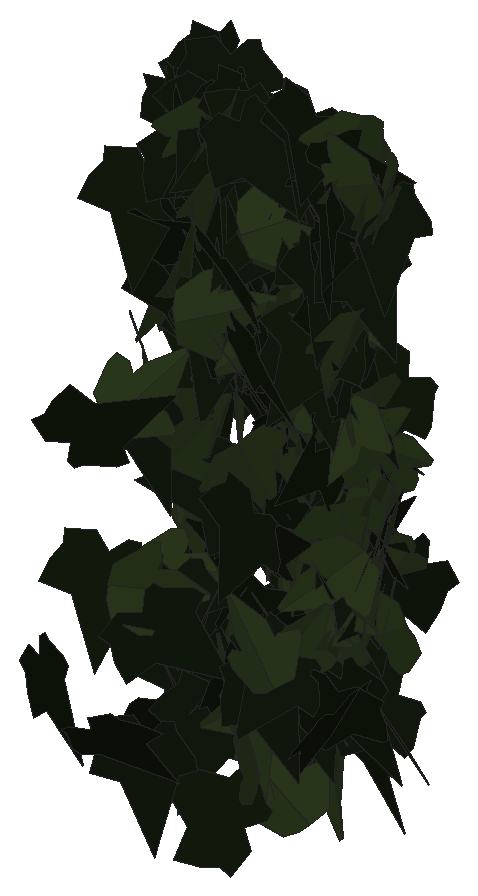
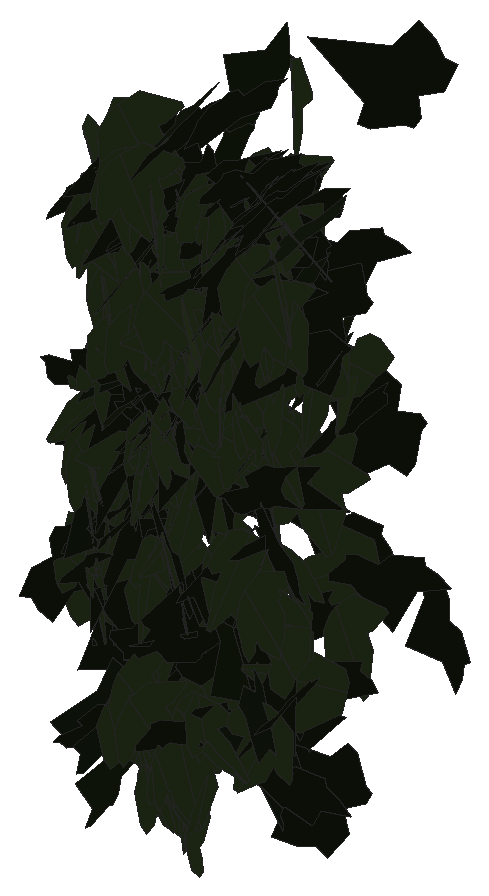
# SketchUp Ruby script. Lengths in inches.
U = 1.inch
M = Sketchup.active_model
def pt(a) = Geom::Point3d.new(a.map { |v| v * U })
def face(e, loops, mat)
  f = e.add_face(loops[0].map { |a| pt(a) })
  loops[1..].each { |l| e.add_face(l.map { |a| pt(a) }).erase! }
  f.material = f.back_material = mat if mat
  f
end
# faces: each face lists its corners as indices into pts; further lists are holes
def faces(e, pts, list, mat = nil) = list.each { |f| face(e, (f[0].is_a?(Array) ? f : [f]).map { |l| l.map { |i| pts[i] } }, mat) }
# xy, xz, yz: faces in a plane at the given z, y or x. An outline is a flat list of corners, or four numbers for a rectangle; further outlines are holes
def ring(l) = l.size == 4 ? [[l[0], l[1]], [l[2], l[1]], [l[2], l[3]], [l[0], l[3]]] : l.each_slice(2).to_a
def flat(e, list, mat, &to3) = list.each { |f| face(e, (f[0].is_a?(Array) ? f : [f]).map { |l| ring(l).map { |u, v| to3.(u, v) } }, mat) }
def xy(e, z, list, mat = nil) = flat(e, list, mat) { |x, y| [x, y, z] }
def xz(e, y, list, mat = nil) = flat(e, list, mat) { |x, z| [x, y, z] }
def yz(e, x, list, mat = nil) = flat(e, list, mat) { |y, z| [x, y, z] }
def lines(e, pts, list) = list.each { |a, b| e.add_line(pt(pts[a]), pt(pts[b])) }
# prism: a flat outline (further loops are holes) pulled along v
def prism(e, loops, v, mat = nil)
  f = face(e, loops, mat); d = Geom::Vector3d.new(v.map { |x| x * U })
  f.pushpull(f.normal.samedirection?(d) ? d.length : -d.length)
end
def box(e, o, s, mat = nil) = prism(e, [[o, [o[0] + s[0], o[1], o[2]], [o[0] + s[0], o[1] + s[1], o[2]], [o[0], o[1] + s[1], o[2]]]], [0, 0, s[2]], mat)
def at(x, y, z, deg = 0) = Geom::Transformation.translation(pt([x, y, z])) * Geom::Transformation.rotation(ORIGIN, Z_AXIS, deg.degrees)
def axes(o, x, y, z) = Geom::Transformation.new([*x, 0, *y, 0, *z, 0, *pt(o).to_a, 1])
def part(name) = M.definitions.add(name)
# library, detail: a bought-in or finely detailed component or shape, given as its bounding box
def library(name, o, s) = part(name).tap { |d| box(d.entities, o, s) }
def detail(e, o, s) = box(e.add_group.entities, o, s)
def put(e, d, t, mat = nil) = e.add_instance(d, t).tap { |i| i.material = mat if mat }
def group(e, t, mat = nil) = e.add_group.tap { |g| g.transformation = t; g.material = mat if mat }.entities
root = M.entities
M.materials.add("efeu1").color = [18, 25, 13]
M.materials.add("efeu2").color = [43, 57, 29]
c1 = part("ivyleaf_9")
p = [[1.54,2.16,1.25],[1.36,2.04,1.19],[-0.21,0.99,0.68],[-0.71,1.11,0.82],[-0.85,0.86,0.67],[-0.8,0.17,0.21],
  [-0.9,-0.01,0.1],[-0.67,-0.16,-0.02],[-0.08,-0.08,-0.05],[-0.03,-0.6,-0.4],[0.65,-0.88,-0.66],[0.83,-0.6,-0.49],
  [1.29,-0.42,-0.43],[1.8125,-0.07,-0.26],[1.21,0.44,0.15]]
faces(c1.entities,p,[[0,1,2,3,4,5,6,7,8,9,10,11,12,13,14]],"efeu1")
c2 = part("ivyleaf_10")
p = [[0,0.5,-0.03],[-0.0625,2.02,-0.43],[-0.19,2.01,-0.46],[-0.54,1.05,-0.29],[-0.52,0.625,-0.18],[-0.83,0.76,-0.28],
  [-1.16,0.64,-0.33],[-1.15,0.33,-0.24],[-0.77,-0.39,0.02],[-0.3,-0.51,0.16],[0.04,-0.48,0.23],[-0.02,2.01,-0.4375],
  [-0.06,2.01,-0.43],[0.04,-0.49,0.23],[0.67,-0.49,0.14],[1.38,0.36,-0.2],[1.375,0.51,-0.24],[0.81,0.65,-0.19],
  [0.62,0.59,-0.15],[0.6,1.09,-0.28],[0.5,1.23,-0.31]]
faces(c2.entities,p,[[0,1,2,3,4,5,6,7,8,9,10],[11,12,0,13,14,15,16,17,18,19,20]],"efeu2")
put(root,c1,axes([15.72,223.31,221.94],[-0.24681,-0.41121,-0.14139],[0.07625,0.11913,-0.47958],[0.4281,-0.25829,0.0039]))
put(root,c1,axes([16.01,224.52,223.05],[-0.47711,0.12724,-0.07858],[0.06987,-0.04261,-0.49326],[-0.13223,-0.48166,0.02288]))
put(root,c1,axes([15.53,224.26,222.49],[0.09405,-0.47818,0.11179],[0.14245,-0.08236,-0.47215],[0.46996,0.12066,0.12075]))
put(root,c2,axes([15.89,224.53,221.48],[-0.07713,-0.43131,0.24088],[-0.01882,-0.24106,-0.43765],[0.49366,-0.07658,0.02096]))
put(root,c2,axes([15.875,223.5,220.27],[0.00494,-0.43053,-0.2542],[0.00579,0.25425,-0.43049],[0.49994,0.00131,0.00749]))
put(root,c2,axes([15.87,224.3125,222.02],[0.28102,-0.40312,-0.09228],[-0.03298,0.08937,-0.49084],[0.41224,0.28196,0.02365]))
put(root,c2,axes([15.9,222.98,216.4375],[0.02403,-0.49077,0.09257],[0.00431,-0.09247,-0.49136],[0.4994,0.02442,-0.00021]))
put(root,c2,axes([15.8,224.23,221.24],[-0.45706,0.1615,-0.12254],[0.11495,-0.0425,-0.48475],[-0.16699,-0.47129,0.00172]))
put(root,c1,axes([15.75,223.69,220.25],[0.29807,-0.33208,-0.22556],[0.14103,-0.1764,0.44609],[-0.37585,-0.32955,-0.01149]))
put(root,c2,axes([15.98,223.55,218.6875],[-0.2588,-0.40903,0.12537],[-0.04354,-0.12058,-0.48328],[0.42559,-0.26106,0.02679]))
put(root,c2,axes([16.15,224.01,219.27],[0.1624,-0.04527,-0.47072],[-0.33712,0.33794,-0.14881],[0.33162,0.36572,0.07924]))
put(root,c1,axes([15.86,222.34,216.99],[-0.29592,-0.35163,-0.19694],[0.1339,0.14468,-0.4595],[0.38014,-0.32469,0.00854]))
put(root,c1,axes([15.62,221.33,215.86],[-0.07203,-0.02713,-0.49404],[0.48828,0.07677,-0.0754],[0.07995,-0.49333,0.01543]))
put(root,c1,axes([15.82,223.68,216.07],[-0.17356,-0.41013,-0.22731],[0.09355,0.20723,-0.44531],[0.45948,-0.19711,0.0048]))
put(root,c2,axes([15.59,223.74,216.01],[0.09983,-0.0186,-0.48958],[0.47012,0.14428,0.09038],[0.13791,-0.47837,0.04629]))
put(root,c1,axes([15.88,224.125,214.86],[-0.35838,-0.23731,-0.25544],[0.22562,0.12144,-0.42936],[0.26582,-0.42301,0.02005]))
put(root,c2,axes([15.91,224.02,217.81],[0.45766,-0.19823,0.03543],[0.03264,-0.01378,-0.49874],[0.19871,0.45882,0.00033]))
put(root,c1,axes([15.77,223.98,220.92],[-0.05537,-0.15535,-0.47202],[0.13167,0.45338,-0.16466],[0.47916,-0.14253,-0.0093]))
put(root,c1,axes([16.13,224.45,218.93],[-0.36383,-0.28923,0.18432],[-0.13053,-0.13172,-0.46434],[0.31716,-0.386,0.02035]))
put(root,c1,axes([15.77,224.36,222.98],[0.17453,-0.42797,-0.19073],[-0.01819,0.19719,-0.45912],[0.4682,0.1672,0.05326]))
put(root,c1,axes([15.87,224.63,223.05],[-0.05741,-0.47814,0.13449],[-0.0107,-0.13416,-0.48155],[0.49658,-0.05816,0.00517]))
put(root,c1,axes([15.78,224.3,223.05],[0.14524,-0.43811,-0.19226],[0.01744,0.20564,-0.45542],[0.47812,0.12559,0.07501]))
put(root,c1,axes([15.83,224.36,215.82],[0.03367,-0.48945,0.09646],[0.00663,-0.09623,-0.49061],[0.49882,0.03432,0.00001]))
put(root,c1,axes([15.72,223.32,214.15],[0.27921,0.40355,-0.09585],[0.05252,0.08021,0.49072],[0.41144,-0.2841,0.00241]))
put(root,c2,axes([16,224.58,217.39],[0.04641,-0.43084,0.24945],[0.08809,-0.23947,-0.42999],[0.48999,0.08386,0.05368]))
put(root,c1,axes([16.15,224.34,215.97],[-0.31423,0.27166,-0.27832],[0.21429,-0.17766,-0.41535],[-0.32456,-0.38031,-0.00478]))
put(root,c2,axes([15.75,224.22,216.5],[-0.2069,-0.07433,0.44907],[0.4482,-0.11935,0.18674],[0.07944,0.47982,0.11602]))
put(root,c2,axes([15.98,224.36,215.57],[-0.46074,0.10604,-0.1627],[0.15514,-0.05102,-0.47258],[-0.11683,-0.48595,0.01411]))
put(root,c1,axes([15.7,223.35,220.99],[0.4058,0.20645,-0.20664],[0.18259,0.09682,0.45529],[0.22801,-0.44498,0.00318]))
put(root,c2,axes([15.93,223,219.4],[-0.28898,0.22288,0.34178],[0.27508,-0.20291,0.36491],[0.30136,0.39894,-0.00535]))
put(root,c1,axes([16.32,223.96,216.53],[0.19746,0.12128,-0.44306],[-0.4272,-0.12879,-0.22564],[-0.16886,0.46766,0.05276]))
put(root,c2,axes([16.14,224.29,221.48],[0.0521,-0.49237,-0.06967],[-0.00268,0.06977,-0.4951],[0.49727,0.05196,0.00463]))
put(root,c1,axes([15.9,224.2,222.79],[0.19559,-0.45805,0.04396],[0.01087,-0.04316,-0.49802],[0.46003,0.19577,-0.00692]))
put(root,c2,axes([16.25,224.41,221.8],[-0.15765,-0.39044,0.26963],[-0.04448,-0.27071,-0.41801],[0.47241,-0.15579,0.05062]))
put(root,c2,axes([15.8,224.07,216.92],[-0.09039,0.00389,-0.49175],[0.45215,-0.19593,-0.08466],[-0.19336,-0.45999,0.0319]))
put(root,c1,axes([16.07,223.97,217.59],[-0.24845,0.30172,0.31183],[0.13853,-0.28537,0.38649],[0.4112,0.27844,0.0582]))
put(root,c2,axes([16.25,223.72,222.73],[-0.07862,-0.41713,0.26423],[-0.00688,-0.26661,-0.42293],[0.49373,-0.07014,0.03618]))
put(root,c2,axes([15.92,224.34,219.57],[-0.11841,0.01429,0.48557],[0.42961,-0.23019,0.11154],[0.22674,0.44363,0.04223]))
put(root,c1,axes([15.93,223.8,221.4],[0.214,-0.41307,0.18325],[0.09205,-0.15866,-0.46514],[0.44242,0.23281,0.00814]))
put(root,c1,axes([16.14,224.43,223.23],[-0.11285,-0.45362,-0.17747],[0.0387,0.17324,-0.46743],[0.48556,-0.11924,-0.00399]))
put(root,c1,axes([16.09,222.66,219.125],[0.12985,-0.45974,-0.14756],[-0.0417,0.14155,-0.47773],[0.48104,0.13638,-0.00158]))
put(root,c1,axes([16.33,224.23,221.47],[-0.36497,-0.34174,-0.00314],[0.0022,0.00224,-0.49999],[0.34174,-0.36498,-0.00014]))
put(root,c2,axes([16.3125,224.12,219.85],[-0.10415,-0.41747,0.2547],[0.07899,-0.27136,-0.41246],[0.48261,-0.04568,0.12248]))
put(root,c1,axes([16.26,224.0625,222.81],[-0.19801,-0.43545,0.14552],[0.01978,-0.16642,-0.47108],[0.45869,-0.1808,0.08313]))
put(root,c1,axes([16.34,224.21,222.14],[-0.16062,-0.28051,0.38146],[-0.11377,-0.36815,-0.31862],[0.45963,-0.18916,0.05444]))
put(root,c1,axes([16.15,223.52,222.46],[0.06827,-0.40449,-0.28588],[0.08286,0.29384,-0.39597],[0.48834,0.00669,0.10715]))
put(root,c1,axes([16.77,223.28,214.93],[-0.05199,0.03645,0.49595],[-0.3914,0.3046,-0.06342],[-0.30676,-0.39483,-0.00314]))
put(root,c2,axes([16.55,223.87,221.83],[-0.29422,-0.38191,0.1326],[-0.04371,-0.13299,-0.48],[0.4019,-0.29405,0.04487]))
put(root,c2,axes([16.79,224.32,219.13],[0.2081,0.00921,-0.45454],[-0.45197,-0.04984,-0.20793],[-0.04914,0.49742,-0.01242]))
put(root,c1,axes([16.21,223.51,222.28],[-0.15281,-0.12418,-0.45959],[0.44452,0.1356,-0.18444],[0.17045,-0.46496,0.06896]))
put(root,c1,axes([16.33,224.4,222.59],[-0.00684,-0.43591,0.24481],[0.01371,-0.24491,-0.4357],[0.49977,0.00075,0.0153]))
put(root,c1,axes([16.35,224.35,222.07],[0.11485,-0.41479,-0.25448],[-0.06772,0.2453,-0.43039],[0.4819,0.13333,0.00016]))
put(root,c1,axes([16.26,224.31,222.5],[0.16438,-0.45492,0.12658],[0.04623,-0.11789,-0.4837],[0.46994,0.17073,0.0033]))
put(root,c1,axes([16.27,224.22,221.39],[0.2331,-0.44224,0.0094],[0.00423,-0.0084,-0.49991],[0.44232,0.23314,-0.00017]))
put(root,c2,axes([16.56,223.81,222.82],[0.09814,-0.48089,-0.09545],[-0.00748,0.09587,-0.49067],[0.49022,0.09773,0.01162]))
put(root,c1,axes([16.4,223.91,219.86],[-0.07315,-0.48565,0.09378],[0.00666,-0.09576,-0.4907],[0.49458,-0.07054,0.02047]))
put(root,c1,axes([16.7,223.88,216.06],[-0.27818,0.25238,-0.33003],[-0.24081,0.22571,0.37558],[0.33856,0.36791,-0.00403]))
put(root,c1,axes([16.31,223.95,219.58],[0.33797,-0.36222,-0.06763],[-0.04741,0.04827,-0.4954],[0.36542,0.34127,-0.00172]))
put(root,c2,axes([16.34,222.18,216.76],[0.02912,0.07811,0.493],[0.22372,0.43942,-0.08284],[-0.44621,0.22541,-0.00935]))
put(root,c2,axes([16.71,224.375,222.61],[-0.38653,-0.30276,0.09449],[-0.06735,-0.06722,-0.49086],[0.30993,-0.3922,0.01119]))
put(root,c2,axes([16.6,223.68,218.72],[0.28316,-0.41171,-0.01763],[-0.00485,0.01806,-0.49965],[0.41206,0.28314,0.00623]))
put(root,c2,axes([16.36,222.07,219.42],[0.26427,0.16431,-0.39136],[0.29627,0.25873,0.30869],[0.30395,-0.39505,0.03939]))
put(root,c2,axes([16.61,224.04,217.66],[-0.09598,-0.37459,-0.31697],[0.09128,0.30371,-0.38656],[0.48214,-0.13207,0.01009]))
put(root,c2,axes([16.44,222.9,218.3],[-0.37516,-0.20924,0.25588],[0.25032,0.07293,0.42664],[-0.21586,0.44822,0.05003]))
put(root,c1,axes([16.4,224.1,217.39],[0.19608,-0.11851,-0.44442],[0.36716,-0.25064,0.22884],[-0.27702,-0.41609,-0.01127]))
put(root,c1,axes([16.84,223.47,215.11],[-0.13393,0.48134,-0.01937],[0.00369,-0.01908,-0.49962],[-0.48171,-0.13398,0.00156]))
put(root,c2,axes([16.72,223.6875,220],[0.1766,-0.35048,-0.3098],[-0.04173,0.31802,-0.38357],[0.46591,0.16133,0.08308]))
put(root,c2,axes([16.54,224.03,219.09],[-0.17371,0.34054,-0.32227],[0.13487,-0.29285,-0.38216],[-0.44904,-0.2197,0.00989]))
put(root,c1,axes([16.55,224.32,222.83],[-0.01228,-0.48452,0.12283],[0.01492,-0.12317,-0.48436],[0.49963,-0.00823,0.01748]))
put(root,c2,axes([16.4,224.41,219.74],[0.34056,-0.01847,0.36562],[0.3656,-0.00837,-0.34097],[0.01872,0.49959,0.00781]))
put(root,c1,axes([16.5,224.58,220.6],[0.05912,-0.37012,0.33094],[0.06448,-0.32473,-0.37469],[0.49229,0.08698,0.00933]))
put(root,c2,axes([16.72,224.38,220.02],[-0.0241,-0.3727,0.33244],[0.06737,-0.33221,-0.36756],[0.49485,0.02708,0.06623]))
put(root,c1,axes([16.52,222.28,216.4],[0.02479,-0.13908,-0.47963],[0.07395,0.47595,-0.13419],[0.49388,-0.06428,0.04417]))
put(root,c2,axes([16.82,224.15,220.27],[0.26066,-0.30579,-0.29757],[-0.07711,0.3092,-0.38529],[0.41965,0.24675,0.11403]))
put(root,c2,axes([16.75,224.33,220.48],[0.00295,-0.38349,0.32082],[0.06983,-0.31737,-0.38],[0.49509,0.04705,0.05168]))
put(root,c1,axes([16.64,224.375,222.08],[-0.07362,-0.4274,0.24882],[0.00432,-0.25211,-0.43177],[0.49453,-0.06142,0.04081]))
put(root,c2,axes([16.83,224.3125,222.5],[0.08456,-0.46465,-0.16417],[0.05693,0.17466,-0.46503],[0.4895,0.05995,0.08245]))
put(root,c2,axes([16.88,223.21,222.29],[0.04951,-0.49611,0.03773],[0.00674,-0.03725,-0.49857],[0.4975,0.04987,0.003]))
put(root,c2,axes([17.13,224.36,215.3],[0.24059,-0.1093,-0.42446],[-0.39882,0.14628,-0.26372],[0.18183,0.46546,-0.0168]))
put(root,c1,axes([16.6875,224.25,217.58],[0.03565,-0.47997,-0.13548],[-0.01024,0.13509,-0.48129],[0.49862,0.03709,-0.00019]))
put(root,c1,axes([17.01,224.02,222.67],[-0.32702,-0.26402,0.27084],[-0.1657,-0.22184,-0.41633],[0.34,-0.36205,0.05759]))
put(root,c2,axes([16.51,224.35,219.51],[-0.15282,0.05447,-0.47295],[0.45619,-0.12532,-0.16183],[-0.13616,-0.48097,-0.01139]))
put(root,c1,axes([17.15,223.74,219.77],[0.18194,0.09994,-0.45487],[-0.40839,-0.20051,-0.2074],[-0.22387,0.447,0.00867]))
put(root,c2,axes([16.95,224.25,215.54],[-0.08038,-0.45398,0.19349],[0.0257,-0.19962,-0.4577],[0.49283,-0.06364,0.05542]))
put(root,c2,axes([16.92,223.99,221.03],[0.11304,-0.47008,0.12747],[0.0496,-0.11906,-0.48308],[0.48452,0.12186,0.01972]))
put(root,c2,axes([16.88,224.21,217.49],[0.09208,-0.43685,0.22513],[0.09929,-0.20779,-0.44381],[0.48131,0.12643,0.04848]))
put(root,c1,axes([16.86,223.18,214.78],[-0.13376,-0.46798,0.11447],[-0.02146,-0.11289,-0.48662],[0.4813,-0.13509,0.01012]))
put(root,c1,axes([17.35,223.13,218.07],[-0.18707,-0.15095,-0.43843],[-0.34116,-0.27537,0.24037],[-0.31403,0.38908,0.00003]))
put(root,c2,axes([17.01,223.74,219.9],[0.27437,-0.37324,-0.18819],[-0.05237,0.19264,-0.45842],[0.4147,0.27127,0.06661]))
put(root,c2,axes([17.02,223.86,222.42],[-0.46302,-0.18806,-0.01578],[0.01454,0.00613,-0.49975],[0.18816,-0.46325,-0.00021]))
put(root,c1,axes([17.11,223.16,215.52],[-0.0798,0.1176,-0.47938],[-0.2755,0.39231,0.1421],[0.40955,0.28682,0.00219]))
put(root,c2,axes([16.88,224.21,220.63],[0.45826,0.01475,0.19945],[0.19939,0.00503,-0.4585],[-0.01553,0.49976,-0.00127]))
put(root,c1,axes([17.13,224.36,221.45],[-0.238,-0.38514,0.21218],[-0.06116,-0.20992,-0.44966],[0.43545,-0.24,0.05281]))
put(root,c1,axes([17.14,223.9,221.95],[-0.28362,-0.40576,0.07012],[-0.03164,-0.06341,-0.49495],[0.41056,-0.28519,0.01029]))
put(root,c2,axes([17.14,224.39,220.9],[0.22407,-0.44663,0.01786],[0.00184,-0.01905,-0.49963],[0.44698,0.22397,-0.00689]))
put(root,c1,axes([16.91,224.14,219.68],[-0.10643,-0.30015,-0.38546],[0.23227,0.31597,-0.31018],[0.42979,-0.24509,0.07217]))
put(root,c2,axes([17.17,223.95,219.95],[-0.1456,-0.04464,0.47624],[0.06474,-0.49508,-0.02662],[0.47393,0.05391,0.14994]))
put(root,c2,axes([17.3,223.78,214.88],[0.04971,0.06466,-0.4933],[-0.25759,-0.4208,-0.08111],[-0.42565,0.2622,-0.00852]))
put(root,c2,axes([17.32,223.04,214.97],[-0.27991,0.38062,-0.16364],[-0.09564,0.1328,0.47246],[0.40312,0.29579,-0.00154]))
put(root,c1,axes([17.13,224.53,215.33],[-0.20232,-0.44769,-0.09297],[0.04165,0.0832,-0.49127],[0.45534,-0.20653,0.00363]))
put(root,c2,axes([17.27,224.375,214.73],[-0.23993,-0.42187,0.12027],[0.02915,-0.15211,-0.47541],[0.4377,-0.22111,0.09758]))
put(root,c2,axes([16.95,222.71,220.63],[0.03725,0.02866,-0.49779],[0.40483,0.28966,0.04697],[0.29107,-0.40654,-0.00163]))
put(root,c2,axes([17.02,224.48,213.81],[0.02949,-0.10279,0.48843],[0.31954,-0.37198,-0.09757],[0.38343,0.31791,0.04375]))
put(root,c1,axes([17.15,224,220.22],[0.29196,-0.27373,-0.29972],[-0.21125,0.21278,-0.40012],[0.3466,0.36027,0.00859]))
put(root,c1,axes([17.09,224.39,220.64],[0.06431,-0.43946,0.22965],[0.01942,-0.22916,-0.44397],[0.49547,0.06602,-0.01241]))
put(root,c2,axes([17.27,224.16,219.65],[0.21908,-0.4479,0.03731],[0.01309,0.04785,0.49753],[-0.44926,-0.21703,0.0327]))
put(root,c1,axes([17.06,223.4,219.62],[0.06929,-0.27636,0.41088],[0.24477,-0.34154,-0.27099],[0.43045,0.2387,0.08796]))
put(root,c2,axes([17.5,224.55,221],[-0.05226,-0.39162,0.30644],[-0.03865,-0.30399,-0.39509],[0.49576,-0.06499,0.0015]))
put(root,c1,axes([17.14,223.94,219.9],[0.24656,-0.42202,0.1054],[0.04981,-0.09297,-0.48875],[0.43212,0.25151,-0.00381]))
put(root,c2,axes([17.43,224.44,214.72],[0.05058,-0.48279,0.1198],[0.04441,-0.11556,-0.48443],[0.49545,0.05965,0.03119]))
put(root,c1,axes([17.12,223.8,215.84],[-0.05117,-0.03999,0.49577],[0.40017,-0.29928,0.01716],[0.29537,0.39854,0.06263]))
put(root,c1,axes([17.61,223.625,218.95],[0.2687,0.0715,-0.41555],[-0.41048,-0.06839,-0.27719],[-0.09648,0.49011,0.02194]))
put(root,c2,axes([17.41,224.59,219.3],[0.13462,-0.38604,0.28784],[0.10783,-0.26712,-0.40868],[0.46931,0.17211,0.01133]))
put(root,c2,axes([17.49,223.95,218.17],[-0.49786,0.03728,-0.02737],[0.02701,-0.00578,-0.49924],[-0.03754,-0.49857,0.00374]))
put(root,c2,axes([17.52,223.92,220.04],[0.02311,-0.49642,0.0551],[0.00331,-0.055,-0.49695],[0.49945,0.02333,0.00074]))
put(root,c1,axes([17.125,224.1,222.3],[0.23128,-0.04539,-0.44096],[0.44225,-0.01056,0.23304],[-0.03047,-0.49782,0.03526]))
put(root,c2,axes([17.54,224.3,217.42],[0.31023,-0.38904,-0.04908],[-0.02548,0.04246,-0.49754],[0.39129,0.31121,0.00652]))
put(root,c2,axes([17.66,223.59,221.77],[-0.4809,0.08265,0.1091],[-0.10724,0.0201,-0.48795],[-0.08505,-0.49271,-0.0016]))
put(root,c1,axes([17.35,224.35,216.96],[-0.07818,0.20933,0.44729],[0.1644,-0.416,0.22342],[0.46568,0.182,-0.00378]))
put(root,c1,axes([17.75,224.26,216.04],[-0.41352,-0.23157,0.15932],[0.14389,0.06905,0.47384],[-0.24145,0.43773,0.00953]))
put(root,c2,axes([17.62,224.46,214.37],[0.00046,-0.45048,0.21696],[0.02404,-0.21669,-0.44997],[0.49942,0.01084,0.02146]))
put(root,c2,axes([17.63,223.95,214.28],[0.14237,-0.45886,-0.1385],[-0.01168,0.14111,-0.47953],[0.47916,0.13978,0.02947]))
put(root,c2,axes([17.62,223.9375,220.02],[0.25512,-0.3483,-0.25219],[-0.01494,0.28587,-0.40994],[0.42975,0.21671,0.13546]))
put(root,c1,axes([17.38,223.12,223.3],[0.15254,-0.38549,-0.27952],[0.01807,0.29799,-0.40109],[0.47582,0.11227,0.10484]))
put(root,c2,axes([17.625,223.95,220.84],[-0.08256,-0.37769,-0.31707],[0.05748,0.31192,-0.38653],[0.48977,-0.10028,-0.00809]))
put(root,c1,axes([17.67,223.59,219.18],[0.15391,0.46586,0.09637],[0.03577,0.08967,-0.49059],[-0.47438,0.15791,-0.00573]))
put(root,c2,axes([17.47,223.7,217.75],[0.24893,-0.22013,0.3736],[0.27247,-0.25572,-0.33221],[0.33733,0.36899,-0.00736]))
put(root,c2,axes([17.76,224.25,219.07],[-0.20207,-0.44577,0.10226],[-0.01846,-0.10376,-0.48877],[0.45698,-0.20131,0.02547]))
put(root,c2,axes([17.64,224.02,220.58],[0.00175,0.01545,-0.49976],[0.13414,0.48142,0.01535],[0.48167,-0.13413,-0.00246]))
put(root,c2,axes([17.82,224.24,217.02],[-0.18389,-0.34918,0.30702],[-0.0325,-0.3197,-0.38306],[0.46382,-0.16084,0.09488]))
put(root,c2,axes([17.63,223.63,221.22],[-0.42049,-0.19327,0.18931],[0.17873,0.06419,0.46253],[-0.20309,0.45665,0.0151]))
put(root,c1,axes([17.67,223.03,216.01],[-0.0423,0.34913,-0.35541],[-0.04613,0.35242,0.35168],[0.49607,0.06254,0.0024]))
put(root,c2,axes([17.82,224.25,222.21],[0.23583,-0.41637,-0.145],[-0.03259,0.14753,-0.47663],[0.43969,0.23426,0.04244]))
put(root,c2,axes([17.83,221.51,222.68],[0.20189,-0.40706,-0.20866],[-0.03817,0.2123,-0.45108],[0.45583,0.19807,0.05465]))
put(root,c1,axes([17.69,223.73,218.97],[-0.04825,0.23141,0.44059],[-0.05675,-0.44233,0.22611],[0.49442,-0.02819,0.06895]))
put(root,c2,axes([17.78,223.62,217.51],[0.04783,-0.17677,-0.46526],[0.1033,0.46075,-0.16444],[0.48687,-0.0804,0.0806]))
put(root,c1,axes([17.67,224.18,223.06],[-0.01702,-0.48075,0.13634],[-0.00216,-0.13634,-0.48105],[0.49971,-0.01696,0.00257]))
put(root,c2,axes([17.87,224.17,217.21],[-0.0067,-0.43236,-0.25105],[0.00621,0.25098,-0.4324],[0.49992,-0.00892,0.002]))
put(root,c1,axes([17.61,224.18,219.38],[0.18402,-0.46313,-0.04064],[-0.00757,0.04072,-0.49828],[0.46484,0.184,0.00798]))
put(root,c2,axes([17.78,223.8,218.4],[-0.28356,-0.40818,0.05461],[0.04191,0.03736,0.49684],[-0.40968,0.28635,0.01302]))
put(root,c1,axes([17.7,224.22,216.44],[0.45787,0.10454,0.17155],[-0.16801,-0.03483,0.46964],[0.11014,-0.48771,0.00323]))
put(root,c1,axes([17.71,223.73,217.93],[-0.10838,-0.22409,0.43363],[0.06031,-0.44694,-0.21589],[0.48437,0.00551,0.12391]))
put(root,c2,axes([17.9,224.21,218.83],[0.02913,-0.40708,-0.28886],[0.01707,0.28999,-0.40695],[0.49886,0.01385,0.03079]))
put(root,c2,axes([17.625,224.55,214.33],[0.34958,-0.12736,0.33403],[0.30903,-0.1272,-0.37192],[0.17971,0.46648,-0.01022]))
put(root,c1,axes([18.24,221.98,214.16],[-0.3512,-0.28902,-0.20767],[-0.15206,-0.14193,0.45468],[-0.32177,0.38252,0.01179]))
put(root,c1,axes([17.79,224.58,218.9],[-0.14913,-0.40264,0.2562],[0.04353,-0.27878,-0.41278],[0.47525,-0.10081,0.11821]))
put(root,c2,axes([17.95,224.42,220.52],[-0.20896,-0.42292,0.16576],[0.01325,-0.18805,-0.4631],[0.45405,-0.18915,0.0898]))
put(root,c1,axes([17.55,223.1,217.55],[0.06206,-0.12165,0.48099],[0.35949,-0.32305,-0.12809],[0.34193,0.36172,0.04737]))
put(root,c2,axes([17.89,224.47,215.18],[-0.09497,-0.39561,0.29065],[0.11255,-0.3057,-0.37932],[0.47782,-0.00662,0.14712]))
put(root,c2,axes([17.57,223.25,221.875],[0.21164,-0.01922,-0.45259],[0.43538,0.14658,0.19737],[0.1251,-0.47764,0.07878]))
put(root,c2,axes([18.02,223.59,218.86],[-0.4084,-0.28302,0.05577],[-0.04558,-0.03215,-0.49688],[0.28484,-0.41093,0.00046]))
put(root,c1,axes([17.74,224.11,223.08],[-0.02606,-0.43006,0.25371],[0.07274,-0.25462,-0.42412],[0.49399,0.0148,0.07583]))
put(root,c1,axes([17.75,224.06,219.18],[0.13784,-0.43963,-0.19423],[-0.02438,0.19541,-0.45959],[0.48001,0.13617,0.03243]))
put(root,c2,axes([18,224.55,222.67],[-0.18338,-0.42992,0.1776],[0.01714,-0.19702,-0.45923],[0.46484,-0.16234,0.08699]))
put(root,c2,axes([17.95,222.43,219.17],[-0.22383,-0.38982,-0.21895],[0.09941,0.19533,-0.4494],[0.43591,-0.24471,-0.00993]))
put(root,c1,axes([17.84,224.2,218.91],[-0.28619,0.19233,0.36209],[0.24644,-0.27221,0.33937],[0.32767,0.37271,0.06101]))
put(root,c2,axes([18.19,224.0625,216.71],[-0.2258,-0.32859,0.30173],[-0.18019,-0.24218,-0.3986],[0.4081,-0.28875,-0.00905]))
put(root,c2,axes([18.07,224.55,215.15],[-0.06153,-0.43725,0.23458],[-0.02899,-0.23281,-0.44154],[0.49535,-0.06794,0.0033]))
put(root,c2,axes([17.96,223.06,214.97],[0.21269,0.44061,-0.1031],[-0.05883,-0.08602,-0.48902],[-0.44867,0.22015,0.01525]))
put(root,c2,axes([17.87,223.92,219.12],[-0.0932,0.15703,0.46546],[0.24037,-0.39859,0.1826],[0.42841,0.25781,-0.0012]))
put(root,c2,axes([18.04,223.25,220.64],[-0.48871,0.1048,-0.01344],[0.01312,-0.00292,-0.49982],[-0.10484,-0.48888,0.0001]))
put(root,c2,axes([17.63,223.78,216.23],[0.03023,-0.00897,0.499],[0.49423,0.07011,-0.02868],[-0.06946,0.49498,0.01311]))
put(root,c2,axes([17.99,224.54,215.56],[-0.01456,-0.38653,0.31683],[0.13432,-0.30833,-0.36998],[0.4814,0.07434,0.11282]))
put(root,c1,axes([17.9,223.84,222.22],[0.08386,-0.15,-0.46954],[-0.02717,0.47416,-0.15632],[0.49217,0.05173,0.07137]))
put(root,c2,axes([18.14,224.375,222.59],[-0.17914,-0.4657,-0.03219],[0.00559,0.03234,-0.49892],[0.46677,-0.17911,-0.00638]))
put(root,c2,axes([18.34,222.99,214],[0.30683,0.212,0.33303],[-0.29107,-0.16346,0.37223],[0.26671,-0.4223,0.0231]))
put(root,c2,axes([18.21,223.96,220.8],[0.29383,-0.32765,-0.2373],[-0.0662,0.25039,-0.42769],[0.3991,0.28276,0.10376]))
put(root,c1,axes([18.04,220.4,216],[-0.30911,-0.22236,-0.32405],[0.253,0.2029,-0.38056],[0.30074,-0.39924,-0.01292]))
put(root,c1,axes([18.33,224.06,219.04],[0.21268,0.00054,-0.45251],[-0.45178,0.02876,-0.2123],[0.0258,0.49917,0.01272]))
put(root,c2,axes([18,223.6,219.09],[-0.34733,0.14582,0.32878],[0.2994,-0.13605,0.37663],[0.1993,0.45851,0.0072]))
put(root,c1,axes([18.0625,223.85,221.68],[0.02028,-0.43995,-0.23671],[-0.01482,0.23627,-0.44041],[0.49937,0.02488,-0.00346]))
put(root,c2,axes([18.33,224.26,220.22],[-0.24881,-0.39539,0.17823],[-0.04273,-0.18212,-0.46369],[0.43159,-0.24597,0.05684]))
put(root,c2,axes([18.3125,224.16,223.09],[-0.16519,-0.4188,0.21752],[0.00104,-0.23078,-0.44355],[0.47192,-0.14609,0.07712]))
put(root,c2,axes([18.3,223.63,216.05],[-0.03898,-0.49237,-0.0778],[-0.00141,0.07815,-0.49385],[0.49848,-0.03829,-0.00748]))
put(root,c1,axes([18.13,223.33,215.73],[-0.02096,-0.42414,-0.26395],[0.01376,0.26359,-0.42465],[0.49937,-0.02507,0.00062]))
put(root,c1,axes([18.13,223.62,222.71],[0.04424,0.09414,-0.48906],[-0.03381,0.49042,0.09134],[0.49689,0.02499,0.04976]))
put(root,c1,axes([18.2,224.29,217.7],[-0.10484,-0.42241,0.24613],[-0.00136,-0.25147,-0.43216],[0.48888,-0.09128,0.05157]))
put(root,c1,axes([18.08,224.39,221.22],[0.09785,-0.45705,0.17758],[0.04438,-0.17208,-0.46735],[0.48832,0.10722,0.00689]))
put(root,c1,axes([18.16,222.52,216.06],[0.08531,-0.43739,-0.22673],[-0.03951,0.22329,-0.44562],[0.49108,0.09395,0.00354]))
put(root,c2,axes([18.35,224.09,222.43],[0.07608,-0.47207,0.14616],[0.05317,-0.1392,-0.47728],[0.49131,0.08816,0.02902]))
put(root,c1,axes([18.23,224.24,219.26],[-0.14172,-0.33185,0.34611],[0.06616,-0.37099,-0.32861],[0.47491,-0.04734,0.14906]))
put(root,c1,axes([18.04,223.57,217.19],[0.09265,-0.21291,0.44281],[0.21016,-0.39014,-0.23156],[0.44413,0.22903,0.0172]))
put(root,c1,axes([18.01,223.98,219.13],[0.45471,-0.07492,0.19397],[0.1906,-0.03627,-0.46082],[0.08311,0.49302,-0.00442]))
put(root,c1,axes([18.35,224.08,218.94],[0.41333,-0.02361,-0.28035],[-0.28066,0.00009,-0.4138],[0.01959,0.49944,-0.01318]))
put(root,c1,axes([18.25,224.09,222.27],[-0.09738,-0.48342,-0.08258],[0.0233,0.07954,-0.49308],[0.48987,-0.09988,0.00703]))
put(root,c2,axes([18.73,223.76,222.67],[-0.161,-0.04405,0.47132],[-0.43955,-0.17089,-0.16612],[0.17572,-0.46782,0.0163]))
put(root,c2,axes([18.28,222.8,216.1],[-0.20284,-0.39835,0.224],[0.11295,0.19377,0.44687],[-0.44283,0.23189,0.01138]))
put(root,c2,axes([18.24,224.32,221.05],[-0.36276,0.17955,-0.29355],[0.24546,-0.16392,-0.40359],[-0.24116,-0.43691,0.03078]))
put(root,c1,axes([18.125,224.55,214.26],[0.26456,-0.38582,0.17649],[0.09551,-0.1485,-0.46779],[0.41338,0.28123,-0.00487]))
put(root,c2,axes([18.32,224.07,218.53],[0.14039,0.44433,0.18127],[0.05779,0.17184,-0.46597],[-0.47639,0.15179,-0.00311]))
put(root,c2,axes([18.56,224.29,217.0625],[-0.43233,-0.21685,-0.12675],[-0.10798,-0.06734,0.48353],[-0.22678,0.44547,0.0114]))
put(root,c1,axes([18.53,224.69,214.9],[-0.27933,-0.31563,0.26899],[-0.10628,-0.259,-0.41427],[0.40085,-0.28861,0.0776]))
put(root,c1,axes([18.43,222.77,216.25],[-0.19034,-0.39781,0.23561],[-0.03928,-0.23996,-0.43689],[0.46068,-0.18483,0.0601]))
put(root,c1,axes([18.31,224.4,222.27],[0.02484,-0.49203,-0.08538],[0.00055,0.08551,-0.49263],[0.49938,0.02438,0.00479]))
put(root,c1,axes([18.32,223.34,220.54],[-0.08975,-0.43749,-0.22483],[0.06007,0.21709,-0.44639],[0.4882,-0.10714,0.01359]))
put(root,c1,axes([18.24,223.82,220.06],[0.47174,-0.16205,-0.03467],[-0.03127,0.01567,-0.49877],[0.16274,0.47275,0.00465]))
put(root,c1,axes([18.31,219.04,216.81],[0.44838,0.21093,0.06683],[0.05889,0.0318,-0.4955],[-0.21329,0.45221,0.00367]))
put(root,c1,axes([18.59,223.38,220.72],[-0.37822,-0.32552,0.03139],[-0.02654,-0.01728,-0.499],[0.32595,-0.37913,-0.00421]))
put(root,c2,axes([18.68,221.98,216.54],[0.39378,0.05832,0.30255],[-0.2972,-0.05768,0.39793],[0.08132,-0.49323,-0.01077]))
put(root,c2,axes([18.27,223.82,219.77],[-0.20119,0.18904,-0.41688],[0.26898,-0.31962,-0.27476],[-0.37036,-0.33482,0.02691]))
put(root,c2,axes([18.43,221.96,215.04],[-0.2778,0.30877,0.27837],[0.18225,-0.21046,0.41532],[0.37365,0.33222,0.00438]))
put(root,c1,axes([18.29,223.54,222.25],[-0.16361,-0.09683,-0.46244],[0.47235,-0.02231,-0.16244],[0.01082,-0.49003,0.09878]))
put(root,c1,axes([18.88,223.36,220.04],[-0.23043,0.28238,0.34229],[-0.22254,0.26013,-0.36443],[-0.38389,-0.3203,0.0058]))
put(root,c1,axes([18.55,224.06,217.53],[0.40007,0.03071,-0.29833],[-0.29705,-0.02785,-0.40123],[-0.04126,0.49828,-0.00403]))
put(root,c2,axes([18.24,223.73,214.27],[0.25377,-0.13205,0.41007],[0.37662,-0.1631,-0.28559],[0.20919,0.45383,0.01669]))
put(root,c1,axes([18.45,224.11,217.65],[-0.11374,-0.48586,0.03169],[-0.005,-0.03138,-0.49899],[0.48687,-0.11383,0.00228]))
put(root,c2,axes([18.16,223.66,216.75],[0.07702,-0.01014,0.49393],[0.49118,0.05521,-0.07546],[-0.05301,0.49684,0.01847]))
put(root,c1,axes([18.4375,224.14,217.35],[-0.16058,-0.39929,-0.25452],[0.08635,0.23956,-0.4303],[0.46557,-0.18215,-0.00798]))
put(root,c2,axes([18.5,223.62,219.22],[0.17079,-0.36206,0.29957],[0.12903,-0.27036,-0.40032],[0.45186,0.21405,0.00108]))
put(root,c1,axes([18.41,223.89,222.13],[-0.00303,-0.39975,0.30032],[0.00276,-0.30033,-0.39974],[0.49998,-0.00076,0.00403]))
put(root,c1,axes([18.5,223.54,220.77],[-0.11157,-0.0821,0.48043],[-0.0454,-0.48896,-0.0941],[0.48527,-0.06462,0.10165]))
put(root,c1,axes([18.41,223.59,221.42],[-0.02021,-0.4669,0.17776],[0.03395,-0.17878,-0.46571],[0.49844,-0.00676,0.03893]))
put(root,c2,axes([18.63,224.05,220.72],[-0.08397,-0.38908,0.3026],[0.01449,-0.30877,-0.393],[0.49268,-0.05724,0.06313]))
put(root,c2,axes([18.65,224.52,221.87],[-0.04476,-0.46038,0.18987],[-0.01911,-0.18891,-0.46255],[0.49763,-0.04867,-0.00068]))
put(root,c1,axes([18.28,218.66,221.11],[0.05085,-0.02854,0.49659],[0.49405,0.06083,-0.0471],[-0.05773,0.49546,0.03439]))
put(root,c2,axes([18.81,223.41,217.45],[0.2576,0.18178,-0.38807],[-0.34095,-0.18736,-0.31408],[-0.25961,0.42644,0.02743]))
put(root,c1,axes([18.46,224.21,217.04],[-0.07386,-0.46327,-0.173],[0.06298,0.16468,-0.46788],[0.49049,-0.0909,0.03402]))
put(root,c1,axes([18.29,221.57,222.4],[0.16607,-0.34568,0.32082],[0.19719,-0.25808,-0.38015],[0.42841,0.25278,0.05061]))
put(root,c2,axes([18.61,224.1,222.29],[0.24135,-0.41323,0.14489],[0.08674,-0.11704,-0.47831],[0.42921,0.25602,0.01519]))
put(root,c1,axes([18.33,224.5,214.92],[0.31051,-0.31971,0.22664],[0.14882,-0.1713,-0.44554],[0.36254,0.34415,-0.01122]))
put(root,c2,axes([18.72,223.875,220.67],[0.13261,-0.48148,0.02424],[0.00564,-0.02359,-0.49941],[0.48206,0.13273,-0.00082]))
put(root,c1,axes([18.49,223.83,219.98],[0.25796,-0.39988,-0.15346],[-0.06151,0.14269,-0.47524],[0.42388,0.26407,0.02443]))
put(root,c2,axes([18.72,224.45,218.42],[0.02131,-0.47621,0.1509],[0.0264,-0.14975,-0.47632],[0.49885,0.02826,0.01876]))
put(root,c1,axes([18.61,223.44,219.12],[0.00425,-0.19127,-0.46195],[0.30759,-0.3632,0.15321],[-0.39417,-0.28548,0.11458]))
put(root,c2,axes([18.79,224.11,218.52],[-0.26551,-0.40112,0.13641],[-0.02652,-0.14493,-0.4778],[0.42285,-0.26096,0.05569]))
put(root,c2,axes([18.75,224.24,221.99],[-0.01629,-0.42893,-0.25643],[0.01259,0.25613,-0.42923],[0.49958,-0.02044,0.00245]))
put(root,c2,axes([18.75,223.41,218.12],[-0.32772,-0.37007,-0.07512],[0.05276,0.05362,-0.49431],[0.37392,-0.33192,0.00391]))
put(root,c2,axes([18.79,223.875,219.59],[-0.14908,-0.47098,-0.07715],[0.01135,0.07731,-0.49386],[0.47712,-0.149,-0.01236]))
put(root,c2,axes([18.5625,223.72,221.19],[0.22089,0.36263,0.26402],[0.14213,0.22254,-0.42459],[-0.42545,0.26262,-0.00477]))
put(root,c2,axes([18.8,224.24,216.88],[0.32683,-0.3535,-0.13499],[-0.06027,0.12746,-0.47971],[0.37357,0.32984,0.0407]))
put(root,c2,axes([18.75,223.44,219.55],[0.45986,0.17025,-0.0977],[-0.09095,-0.03573,-0.49036],[-0.17395,0.46876,-0.00189]))
put(root,c1,axes([18.93,223.86,217.56],[-0.1583,0.19621,-0.43179],[-0.31954,0.29226,0.24996],[0.35048,0.35509,0.03287]))
put(root,c1,axes([18.93,223.06,215.79],[0.2286,0.22847,-0.3815],[-0.26263,-0.27679,-0.32313],[-0.35884,0.34812,-0.00654]))
put(root,c1,axes([18.91,224.41,219.65],[-0.45331,-0.21092,-0.00529],[0.00413,0.00366,-0.49997],[0.21094,-0.45332,-0.00158]))
put(root,c2,axes([18.83,224.27,217.8125],[0.25173,-0.41495,-0.1202],[-0.03095,0.12144,-0.48404],[0.4309,0.25113,0.03546]))
put(root,c2,axes([18.9375,224.22,217.1],[-0.18405,-0.40396,0.23009],[-0.07738,-0.21739,-0.44357],[0.45841,-0.19888,0.0175]))
put(root,c2,axes([18.875,224.02,217.53],[0.30173,-0.34807,-0.19445],[-0.06699,0.19613,-0.45502],[0.39303,0.30063,0.07172]))
put(root,c2,axes([18.85,224.14,218.05],[0.29452,-0.39782,-0.07068],[-0.03177,0.0644,-0.49482],[0.4028,0.29595,0.01266]))
put(root,c1,axes([18.71,221.64,218.87],[-0.05541,-0.42456,0.25822],[-0.01664,-0.25808,-0.42792],[0.49664,-0.05601,0.01447]))
put(root,c2,axes([19.18,223.91,216.42],[-0.2598,-0.01663,0.42688],[-0.41238,-0.12072,-0.25567],[0.11157,-0.48492,0.049]))
put(root,c2,axes([18.8,224.11,218.22],[0.21934,-0.41195,0.1794],[0.07641,-0.16253,-0.46663],[0.44278,0.23212,-0.00835]))
put(root,c1,axes([18.71,224.29,222.21],[-0.04822,-0.49395,-0.06076],[-0.00273,0.06131,-0.49622],[0.49766,-0.04752,-0.00861]))
put(root,c2,axes([18.87,224.16,222.58],[0.28162,-0.41302,-0.01033],[-0.00422,0.00962,-0.49989],[0.41313,0.28164,0.00193]))
put(root,c1,axes([19.07,222.8125,215.65],[-0.15684,0.4541,-0.13855],[0.03979,-0.13283,-0.48039],[-0.47309,-0.16171,0.00553]))
put(root,c2,axes([18.9375,223.31,220.91],[0.00004,-0.4848,0.12235],[0.01119,-0.12232,-0.48468],[0.49987,0.00278,0.01084]))
put(root,c2,axes([18.77,224.2,216.92],[0.11847,-0.318,0.3672],[0.20473,-0.31007,-0.33458],[0.44051,0.22963,0.05674]))
put(root,c1,axes([18.73,223.72,221.73],[0.06695,-0.44719,-0.2134],[0.00384,0.2158,-0.45102],[0.49548,0.05875,0.03233]))
put(root,c1,axes([18.7,223.47,215.68],[-0.11702,-0.0561,-0.48287],[0.42247,0.23396,-0.12956],[0.24047,-0.43831,-0.00736]))
put(root,c1,axes([18.83,221.24,221.62],[0.40719,-0.23229,-0.17389],[-0.14947,0.08892,-0.46878],[0.24871,0.43375,0.00297]))
put(root,c2,axes([18.87,223.75,219.07],[-0.18714,-0.22318,-0.40641],[0.25196,0.31896,-0.29117],[0.38923,-0.31377,-0.00691]))
put(root,c1,axes([19.07,224.59,216.98],[-0.03395,-0.04023,-0.49722],[0.13767,-0.47977,0.02942],[-0.47947,-0.13491,0.04365]))
